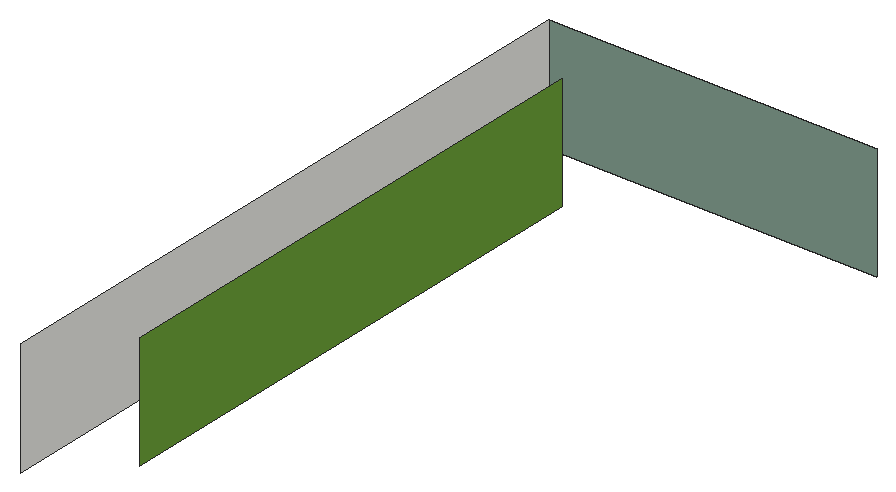
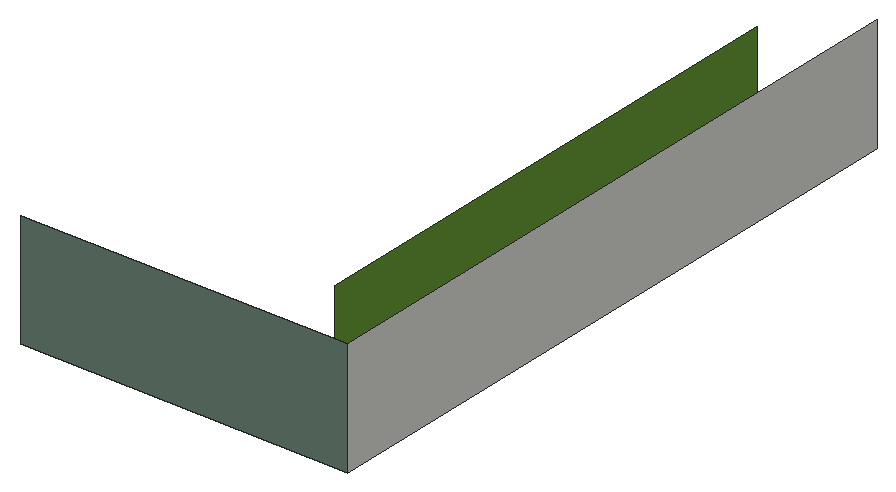
# SketchUp Ruby script. Lengths in inches.
U = 1.inch
M = Sketchup.active_model
def pt(a) = Geom::Point3d.new(a.map { |v| v * U })
def face(e, loops, mat)
  f = e.add_face(loops[0].map { |a| pt(a) })
  loops[1..].each { |l| e.add_face(l.map { |a| pt(a) }).erase! }
  f.material = f.back_material = mat if mat
  f
end
# faces: each face lists its corners as indices into pts; further lists are holes
def faces(e, pts, list, mat = nil) = list.each { |f| face(e, (f[0].is_a?(Array) ? f : [f]).map { |l| l.map { |i| pts[i] } }, mat) }
# xy, xz, yz: faces in a plane at the given z, y or x. An outline is a flat list of corners, or four numbers for a rectangle; further outlines are holes
def ring(l) = l.size == 4 ? [[l[0], l[1]], [l[2], l[1]], [l[2], l[3]], [l[0], l[3]]] : l.each_slice(2).to_a
def flat(e, list, mat, &to3) = list.each { |f| face(e, (f[0].is_a?(Array) ? f : [f]).map { |l| ring(l).map { |u, v| to3.(u, v) } }, mat) }
def xy(e, z, list, mat = nil) = flat(e, list, mat) { |x, y| [x, y, z] }
def xz(e, y, list, mat = nil) = flat(e, list, mat) { |x, z| [x, y, z] }
def yz(e, x, list, mat = nil) = flat(e, list, mat) { |y, z| [x, y, z] }
def lines(e, pts, list) = list.each { |a, b| e.add_line(pt(pts[a]), pt(pts[b])) }
# prism: a flat outline (further loops are holes) pulled along v
def prism(e, loops, v, mat = nil)
  f = face(e, loops, mat); d = Geom::Vector3d.new(v.map { |x| x * U })
  f.pushpull(f.normal.samedirection?(d) ? d.length : -d.length)
end
def box(e, o, s, mat = nil) = prism(e, [[o, [o[0] + s[0], o[1], o[2]], [o[0] + s[0], o[1] + s[1], o[2]], [o[0], o[1] + s[1], o[2]]]], [0, 0, s[2]], mat)
def at(x, y, z, deg = 0) = Geom::Transformation.translation(pt([x, y, z])) * Geom::Transformation.rotation(ORIGIN, Z_AXIS, deg.degrees)
def axes(o, x, y, z) = Geom::Transformation.new([*x, 0, *y, 0, *z, 0, *pt(o).to_a, 1])
def part(name) = M.definitions.add(name)
# library, detail: a bought-in or finely detailed component or shape, given as its bounding box
def library(name, o, s) = part(name).tap { |d| box(d.entities, o, s) }
def detail(e, o, s) = box(e.add_group.entities, o, s)
def put(e, d, t, mat = nil) = e.add_instance(d, t).tap { |i| i.material = mat if mat }
def group(e, t, mat = nil) = e.add_group.tap { |g| g.transformation = t; g.material = mat if mat }.entities
root = M.entities
M.materials.add("[Color H08]").color = [130, 158, 143]
M.materials.add("[Grass Dark Green]").color = [106, 157, 55]
xz(root,85.1875,[[21.01,9,42.01,16.375]],"[Color H08]")
yz(root,21.01,[[42.875,9,85.1875,16.375]])
yz(root,25.26,[[47.13,9,80.93,16.375]],"[Grass Dark Green]")
